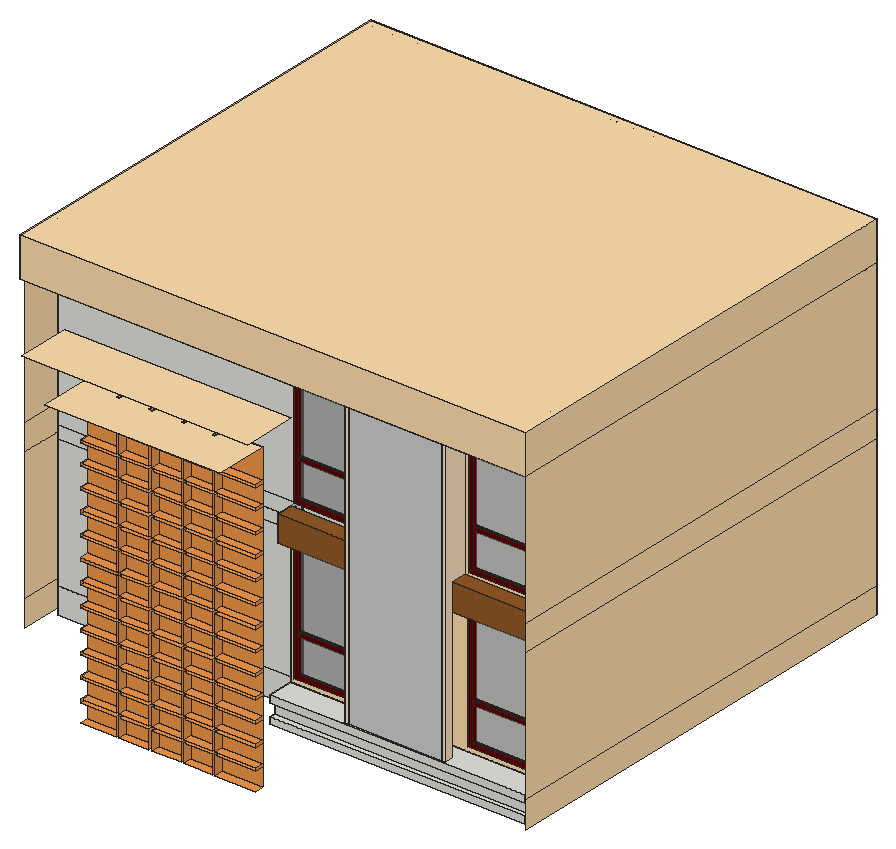
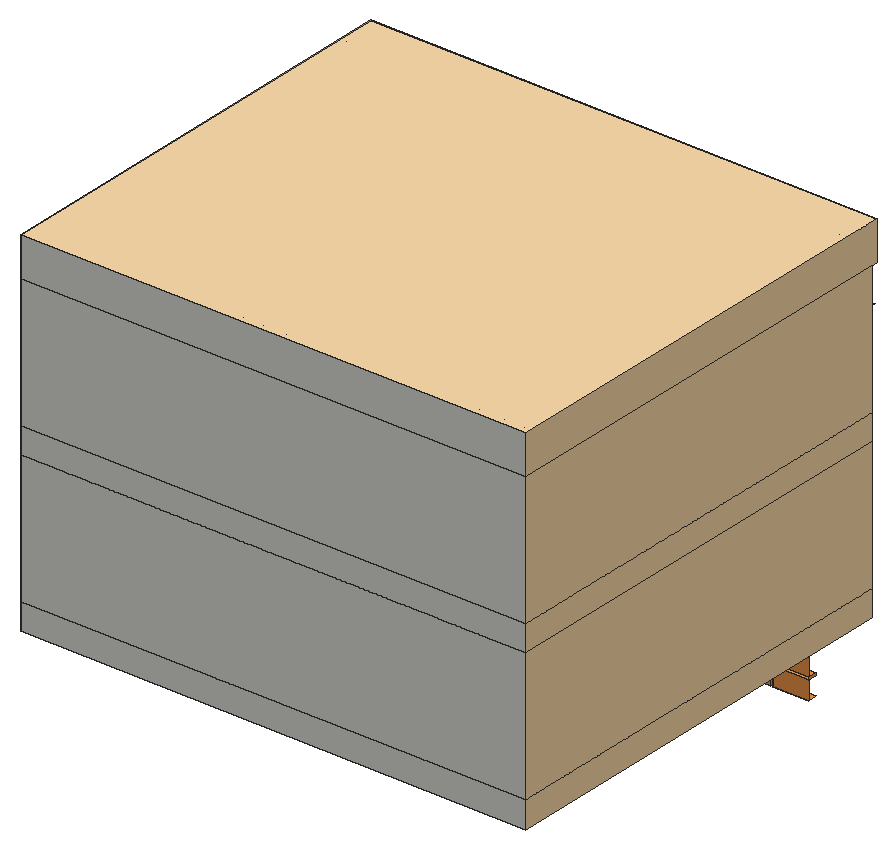
# SketchUp Ruby script. Lengths in inches.
U = 1.inch
M = Sketchup.active_model
def pt(a) = Geom::Point3d.new(a.map { |v| v * U })
def face(e, loops, mat)
  f = e.add_face(loops[0].map { |a| pt(a) })
  loops[1..].each { |l| e.add_face(l.map { |a| pt(a) }).erase! }
  f.material = f.back_material = mat if mat
  f
end
# faces: each face lists its corners as indices into pts; further lists are holes
def faces(e, pts, list, mat = nil) = list.each { |f| face(e, (f[0].is_a?(Array) ? f : [f]).map { |l| l.map { |i| pts[i] } }, mat) }
# xy, xz, yz: faces in a plane at the given z, y or x. An outline is a flat list of corners, or four numbers for a rectangle; further outlines are holes
def ring(l) = l.size == 4 ? [[l[0], l[1]], [l[2], l[1]], [l[2], l[3]], [l[0], l[3]]] : l.each_slice(2).to_a
def flat(e, list, mat, &to3) = list.each { |f| face(e, (f[0].is_a?(Array) ? f : [f]).map { |l| ring(l).map { |u, v| to3.(u, v) } }, mat) }
def xy(e, z, list, mat = nil) = flat(e, list, mat) { |x, y| [x, y, z] }
def xz(e, y, list, mat = nil) = flat(e, list, mat) { |x, z| [x, y, z] }
def yz(e, x, list, mat = nil) = flat(e, list, mat) { |y, z| [x, y, z] }
def lines(e, pts, list) = list.each { |a, b| e.add_line(pt(pts[a]), pt(pts[b])) }
# prism: a flat outline (further loops are holes) pulled along v
def prism(e, loops, v, mat = nil)
  f = face(e, loops, mat); d = Geom::Vector3d.new(v.map { |x| x * U })
  f.pushpull(f.normal.samedirection?(d) ? d.length : -d.length)
end
def box(e, o, s, mat = nil) = prism(e, [[o, [o[0] + s[0], o[1], o[2]], [o[0] + s[0], o[1] + s[1], o[2]], [o[0], o[1] + s[1], o[2]]]], [0, 0, s[2]], mat)
def at(x, y, z, deg = 0) = Geom::Transformation.translation(pt([x, y, z])) * Geom::Transformation.rotation(ORIGIN, Z_AXIS, deg.degrees)
def axes(o, x, y, z) = Geom::Transformation.new([*x, 0, *y, 0, *z, 0, *pt(o).to_a, 1])
def part(name) = M.definitions.add(name)
# library, detail: a bought-in or finely detailed component or shape, given as its bounding box
def library(name, o, s) = part(name).tap { |d| box(d.entities, o, s) }
def detail(e, o, s) = box(e.add_group.entities, o, s)
def put(e, d, t, mat = nil) = e.add_instance(d, t).tap { |i| i.material = mat if mat }
def group(e, t, mat = nil) = e.add_group.tap { |g| g.transformation = t; g.material = mat if mat }.entities
root = M.entities
M.materials.add("[0012_Bisque]").color = [255, 228, 196]
M.materials.add("[0033_NavajoWhite]").color = [255, 222, 173]
M.materials.add("[Carrera Marble]").color = [207, 207, 207]
M.materials.add("[Color A08]").color = [102, 0, 0]
M.materials.add("[Translucent Glass Gray]").color = [128, 128, 128]
M.materials["[Translucent Glass Gray]"].alpha = 0.5
M.materials.add("[Wood Floor Parquet]").color = [145, 89, 39]
M.materials.add("[Wood OSB]").color = [240, 151, 74]
c1 = part("Group\#2")
xy(c1.entities,0,[[0,0,28.5,3]],"[Color A08]")
xy(c1.entities,1.97,[[1.97,0,26.53,3]],"[Color A08]")
xy(c1.entities,16.48,[[1.97,0,26.53,3]],"[Color A08]")
xy(c1.entities,17.92,[[1.97,0,26.53,3]],"[Color A08]")
xy(c1.entities,49.78,[[1.97,0,26.53,3]],"[Color A08]")
xy(c1.entities,51.75,[[0,0,28.5,3]],"[Color A08]")
xz(c1.entities,0,[[[0,0,28.5,51.75],[1.97,1.97,1.97,49.78,26.53,49.78,26.53,17.92,1.97,17.92,1.97,16.48,26.53,16.48,26.53,1.97]]],"[Color A08]")
xz(c1.entities,3,[[[0,0,28.5,51.75],[1.97,1.97,26.53,1.97,26.53,16.48,1.97,16.48,1.97,17.92,26.53,17.92,26.53,49.78,1.97,49.78]]],"[Color A08]")
xz(c1.entities,3,[[1.97,1.97,26.53,16.48],[1.97,17.92,26.53,49.78]],"[Translucent Glass Gray]")
yz(c1.entities,0,[[0,0,3,51.75]],"[Color A08]")
yz(c1.entities,1.97,[[0,1.97,3,16.48],[0,16.48,3,17.92],[0,17.92,3,49.78]],"[Color A08]")
yz(c1.entities,26.53,[[0,1.97,3,16.48],[0,17.92,3,49.78]],"[Color A08]")
yz(c1.entities,28.5,[[0,0,3,51.75]],"[Color A08]")
xy(root,355.36,[[104.2,92.4375,136.74,100.4375],[139.19,92.4375,165.875,100.4375],[169.17,92.4375,195.99,100.4375],[198.13,92.4375,224.24,100.4375],[226.62,92.4375,263.87,100.4375]],"[Wood OSB]")
xy(root,372.03,[[104.2,92.4375,136.74,100.4375],[139.19,92.4375,165.875,100.4375],[169.17,92.4375,195.99,100.4375],[198.13,92.4375,224.24,100.4375],[226.62,92.4375,263.87,100.4375]],"[Wood OSB]")
xy(root,374.67,[[104.2,92.4375,136.74,100.4375],[139.19,92.4375,165.875,100.4375],[169.17,92.4375,195.99,100.4375],[198.13,92.4375,224.24,100.4375],[226.62,92.4375,263.87,100.4375]],"[Wood OSB]")
xy(root,391.34,[[104.2,92.4375,136.74,100.4375],[139.19,92.4375,165.875,100.4375],[169.17,92.4375,195.99,100.4375],[198.13,92.4375,224.24,100.4375],[226.62,92.4375,263.87,100.4375]],"[Wood OSB]")
xy(root,393.98,[[104.2,92.4375,136.74,100.4375],[139.19,92.4375,165.875,100.4375],[169.17,92.4375,195.99,100.4375],[198.13,92.4375,224.24,100.4375],[226.62,92.4375,263.87,100.4375]],"[Wood OSB]")
xy(root,410.65,[[104.2,92.4375,136.74,100.4375],[139.19,92.4375,165.875,100.4375],[169.17,92.4375,195.99,100.4375],[198.13,92.4375,224.24,100.4375],[226.62,92.4375,263.87,100.4375]],"[Wood OSB]")
xy(root,413.3,[[104.2,92.4375,136.74,100.4375],[139.19,92.4375,165.875,100.4375],[169.17,92.4375,195.99,100.4375],[198.13,92.4375,224.24,100.4375],[226.62,92.4375,263.87,100.4375]],"[Wood OSB]")
xy(root,419.04,[[302.01,100.4375,501.57,106.4375]])
xy(root,424.5,[[295.25,106.4375,521.3125,465.125]])
xy(root,426.125,[[289.0625,77,521.3125,100.4375]])
xy(root,429.97,[[104.2,92.4375,136.74,100.4375],[139.19,92.4375,165.875,100.4375],[169.17,92.4375,195.99,100.4375],[198.13,92.4375,224.24,100.4375],[226.62,92.4375,263.87,100.4375]],"[Wood OSB]")
xy(root,432.1875,[[289.0625,77,521.3125,82.1875],[289.0625,82.1875,521.3125,100.4375]])
xy(root,432.61,[[104.2,92.4375,136.74,100.4375],[139.19,92.4375,165.875,100.4375],[169.17,92.4375,195.99,100.4375],[198.13,92.4375,224.24,100.4375],[226.62,92.4375,263.87,100.4375]],"[Wood OSB]")
xy(root,443.4375,[[289.0625,77,521.3125,82.1875],[289.0625,82.1875,521.3125,100.4375]])
xy(root,449.28,[[104.2,92.4375,136.74,100.4375],[139.19,92.4375,165.875,100.4375],[169.17,92.4375,195.99,100.4375],[198.13,92.4375,224.24,100.4375],[226.62,92.4375,263.87,100.4375]],"[Wood OSB]")
xy(root,450.125,[[289.0625,77,355.82,77,355.82,92.4375,359.53,92.4375,359.53,85.8125,448.02,85.8125,448.02,77,521.3125,77,521.3125,100.4375,289.0625,100.4375],[359.53,77,444.31,78.5625],[359.53,78.5625,444.31,85.8125],[71.75,106.4375,289.0625,465.125],[295.0625,106.4375,295.25,465.125],
  [295.25,106.4375,521.3125,465.125]])
xy(root,450.125,[[355.82,77,359.53,78.5625],[444.31,77,448.02,78.5625],[444.31,78.5625,448.02,85.8125]],"[0012_Bisque]")
xy(root,451.92,[[104.2,92.4375,136.74,100.4375],[139.19,92.4375,165.875,100.4375],[169.17,92.4375,195.99,100.4375],[198.13,92.4375,224.24,100.4375],[226.62,92.4375,263.87,100.4375]],"[Wood OSB]")
xy(root,453.93,[[451.2,100.4375,514.83,106.4375]])
xy(root,453.97,[[291.92,100.4375,351.54,106.4375]])
xy(root,468.59,[[104.2,92.4375,136.74,100.4375],[139.19,92.4375,165.875,100.4375],[169.17,92.4375,195.99,100.4375],[198.13,92.4375,224.24,100.4375],[226.62,92.4375,263.87,100.4375]],"[Wood OSB]")
xy(root,471.23,[[104.2,92.4375,136.74,100.4375],[139.19,92.4375,165.875,100.4375],[169.17,92.4375,195.99,100.4375],[198.13,92.4375,224.24,100.4375],[226.62,92.4375,263.87,100.4375]],"[Wood OSB]")
xy(root,487.9,[[104.2,92.4375,136.74,100.4375],[136.74,92.4375,139.19,100.4375],[139.19,92.4375,165.875,100.4375],[169.17,92.4375,195.99,100.4375],[198.13,92.4375,224.24,100.4375],
  [226.62,92.4375,263.87,100.4375]],"[Wood OSB]")
xy(root,490.55,[[104.2,92.4375,136.74,100.4375],[136.74,92.4375,139.19,100.4375],[139.19,92.4375,165.875,100.4375],[169.17,92.4375,195.99,100.4375],[198.13,92.4375,224.24,100.4375],
  [226.62,92.4375,263.87,100.4375]],"[Wood OSB]")
xy(root,507.22,[[104.2,92.4375,136.74,100.4375],[139.19,92.4375,165.875,100.4375],[169.17,92.4375,195.99,100.4375],[198.13,92.4375,224.24,100.4375],[226.62,92.4375,263.87,100.4375]],"[Wood OSB]")
xy(root,509.86,[[104.2,92.4375,136.74,100.4375],[139.19,92.4375,165.875,100.4375],[169.17,92.4375,195.99,100.4375],[198.13,92.4375,224.24,100.4375],[226.62,92.4375,263.87,100.4375]],"[Wood OSB]")
xy(root,526.53,[[104.2,92.4375,136.74,100.4375],[139.19,92.4375,165.875,100.4375],[169.17,92.4375,195.99,100.4375],[198.13,92.4375,224.24,100.4375],[226.62,92.4375,263.87,100.4375]],"[Wood OSB]")
xy(root,529.17,[[104.2,92.4375,136.74,100.4375],[139.19,92.4375,165.875,100.4375],[169.17,92.4375,195.99,100.4375],[198.13,92.4375,224.24,100.4375],[226.62,92.4375,263.87,100.4375]],"[Wood OSB]")
xy(root,545.84,[[104.2,92.4375,136.74,100.4375],[139.19,92.4375,165.875,100.4375],[169.17,92.4375,195.99,100.4375],[198.13,92.4375,224.24,100.4375],[226.62,92.4375,263.87,100.4375]],"[Wood OSB]")
xy(root,548.48,[[104.2,92.4375,136.74,100.4375],[139.19,92.4375,165.875,100.4375],[169.17,92.4375,195.99,100.4375],[198.13,92.4375,224.24,100.4375],[226.62,92.4375,263.87,100.4375]],"[Wood OSB]")
xy(root,565.15,[[104.2,92.4375,136.74,100.4375],[139.19,92.4375,165.875,100.4375],[169.17,92.4375,195.99,100.4375],[198.13,92.4375,224.24,100.4375],[226.62,92.4375,263.87,100.4375]],"[Wood OSB]")
xy(root,566.47,[[291.92,100.4375,351.54,106.4375]])
xy(root,567.56,[[451.2,100.4375,514.83,106.4375]])
xy(root,567.8,[[104.2,92.4375,136.74,100.4375],[139.19,92.4375,165.875,100.4375],[169.17,92.4375,195.99,100.4375],[198.13,92.4375,224.24,100.4375],[226.62,92.4375,263.87,100.4375]],"[Wood OSB]")
xy(root,570.125,[[295.0625,106.4375,295.25,465.125]])
xy(root,570.125,[[355.82,85.8125,359.53,92.4375]],"[0012_Bisque]")
xy(root,570.125,[[289.0625,85.8125,289.0625,100.4375,521.3125,100.4375,521.3125,85.8125,359.53,85.8125,359.53,92.4375,355.82,92.4375,355.82,85.8125]],"[Wood Floor Parquet]")
xy(root,581.3125,[[71.75,106.4375,289.0625,465.125]])
xy(root,584.47,[[104.2,92.4375,136.74,100.4375],[139.19,92.4375,165.875,100.4375],[169.17,92.4375,195.99,100.4375],[198.13,92.4375,224.24,100.4375],[226.62,92.4375,263.87,100.4375]],"[Wood OSB]")
xy(root,587.11,[[104.2,92.4375,136.74,100.4375],[139.19,92.4375,165.875,100.4375],[169.17,92.4375,195.99,100.4375],[198.13,92.4375,224.24,100.4375],[226.62,92.4375,263.87,100.4375]],"[Wood OSB]")
xy(root,594.125,[[71.75,106.4375,289.0625,465.125],[295.0625,106.4375,521.3125,465.125]])
xy(root,594.125,[[289.0625,85.8125,355.82,100.4375],[355.82,85.8125,359.53,100.4375],[359.53,85.8125,444.31,100.4375],[444.31,85.8125,448.02,100.4375],[448.02,85.8125,521.3125,100.4375]],"[Wood Floor Parquet]")
xy(root,596.59,[[451.48,100.4375,515.23,106.4375]])
xy(root,597.4375,[[292.08,100.4375,351.27,106.4375]])
xy(root,603.78,[[104.2,92.4375,136.74,100.4375],[139.19,92.4375,165.875,100.4375],[169.17,92.4375,195.99,100.4375],[198.13,92.4375,224.24,100.4375],[226.62,92.4375,263.87,100.4375]],"[Wood OSB]")
xy(root,606.42,[[104.2,92.4375,136.74,100.4375],[139.19,92.4375,165.875,100.4375],[169.17,92.4375,195.99,100.4375],[198.13,92.4375,224.24,100.4375],[226.62,92.4375,263.87,100.4375]],"[Wood OSB]")
xy(root,633.42,[[104.2,51.6875,104.2,100.4375,136.74,100.4375,136.74,92.4375,139.19,92.4375,139.19,100.4375,165.875,100.4375,165.875,92.4375,169.17,92.4375,169.17,100.4375,195.99,100.4375,195.99,92.4375,198.13,92.4375,198.13,100.4375,224.24,100.4375,224.24,92.4375,226.62,92.4375,226.62,100.4375,263.87,100.4375,263.87,51.6875]],"[0033_NavajoWhite]")
xy(root,633.42,[[136.74,92.4375,139.19,100.4375],[165.875,92.4375,169.17,100.4375],[195.99,92.4375,198.13,100.4375],[224.24,92.4375,226.62,100.4375]],"[Wood OSB]")
xy(root,665.86,[[82.77,51.6875,289.0625,100.4375]],"[0033_NavajoWhite]")
xy(root,710.4,[[359.53,78.5625,444.31,100.4375]])
xy(root,711.0625,[[292.08,100.4375,351.27,106.4375]])
xy(root,711.15,[[451.48,100.4375,515.23,106.4375]])
xy(root,714.125,[[[521.3125,71.3125,521.3125,100.4375,289.0625,100.4375,289.0625,465.125,71.75,465.125,71.75,106.4375,289.0625,106.4375,289.0625,100.4375,71.75,100.4375,71.75,77,65.75,77,65.75,471.125,527.3125,471.125,527.3125,71.3125],[295.0625,106.4375,521.3125,465.125]]])
xy(root,714.125,[[355.82,78.5625,448.02,100.4375]],"[0012_Bisque]")
xy(root,714.125,[[65.75,71.3125,65.75,77,71.75,77,71.75,100.4375,355.82,100.4375,355.82,78.5625,448.02,78.5625,448.02,100.4375,521.3125,100.4375,521.3125,71.3125]],"[0033_NavajoWhite]")
xy(root,745.125,[[71.75,106.4375,289.0625,465.125],[295.0625,106.4375,521.3125,465.125]])
xy(root,750.125,[[65.75,71.3125,527.3125,471.125]],"[0033_NavajoWhite]")
xz(root,71.3125,[[65.75,714.125,527.3125,750.125]],"[0033_NavajoWhite]")
xz(root,77,[[289.0625,426.125,521.3125,432.1875],[289.0625,443.4375,521.3125,450.125]])
xz(root,78.5625,[[355.82,450.125,359.53,450.125,359.53,710.4,444.31,710.4,444.31,450.125,448.02,450.125,448.02,714.125,355.82,714.125]],"[0012_Bisque]")
xz(root,78.5625,[[359.53,450.125,444.31,710.4]],"[Carrera Marble]")
xz(root,82.1875,[[289.0625,432.1875,521.3125,443.4375]])
xz(root,85.8125,[[359.53,450.125,444.31,570.125],[359.53,570.125,444.31,594.125]])
xz(root,85.8125,[[444.31,450.125,448.02,570.125]],"[0012_Bisque]")
xz(root,85.8125,[[289.0625,570.125,355.82,594.125],[355.82,570.125,359.53,594.125],[444.31,570.125,448.02,594.125],[448.02,570.125,521.3125,594.125]],"[Wood Floor Parquet]")
xz(root,92.4375,[[355.82,450.125,359.53,570.125]],"[0012_Bisque]")
xz(root,92.4375,[[104.2,487.9,139.19,490.55]],"[Wood OSB]")
xz(root,100.4375,[[289.0625,426.125,521.3125,432.1875],[289.0625,443.4375,521.3125,450.125],[355.82,590.41,448.02,594.125],[355.82,714.125,448.02,717.84]])
xz(root,100.4375,[[355.82,594.125,355.82,714.125,448.02,714.125,448.02,594.125,444.31,594.125,444.31,710.4,359.53,710.4,359.53,594.125]],"[0012_Bisque]")
xz(root,100.4375,[[[289.0625,450.125,521.3125,570.125],[451.2,453.93,514.83,567.56],[291.92,453.97,351.54,566.47]],[[448.02,594.125,521.3125,714.125],[451.48,596.59,515.23,711.15]]],"[0033_NavajoWhite]")
xz(root,100.4375,[[104.2,355.36,136.74,372.03],[139.19,355.36,165.875,372.03],[169.17,355.36,195.99,372.03],[198.13,355.36,224.24,372.03],[226.62,355.36,263.87,372.03],
  [104.2,374.67,136.74,391.34],[139.19,374.67,165.875,391.34],[169.17,374.67,195.99,391.34],[198.13,374.67,224.24,391.34],[226.62,374.67,263.87,391.34],
  [104.2,393.98,136.74,410.65],[139.19,393.98,165.875,410.65],[169.17,393.98,195.99,410.65],[198.13,393.98,224.24,410.65],[226.62,393.98,263.87,410.65],
  [104.2,413.3,136.74,429.97],[139.19,413.3,165.875,429.97],[169.17,413.3,195.99,429.97],[198.13,413.3,224.24,429.97],[226.62,413.3,263.87,429.97],
  [104.2,432.61,136.74,449.28],[139.19,432.61,165.875,449.28],[169.17,432.61,195.99,449.28],[198.13,432.61,224.24,449.28],[226.62,432.61,263.87,449.28],
  [104.2,451.92,136.74,468.59],[139.19,451.92,165.875,468.59],[169.17,451.92,195.99,468.59],[198.13,451.92,224.24,468.59],[226.62,451.92,263.87,468.59],
  [104.2,471.23,136.74,487.9],[139.19,471.23,165.875,487.9],[169.17,471.23,195.99,487.9],[198.13,471.23,224.24,487.9],[226.62,471.23,263.87,487.9],
  [104.2,490.55,136.74,507.22],[139.19,490.55,165.875,507.22],[169.17,490.55,195.99,507.22],[198.13,490.55,224.24,507.22],[226.62,490.55,263.87,507.22],
  [104.2,509.86,136.74,526.53],[139.19,509.86,165.875,526.53],[169.17,509.86,195.99,526.53],[198.13,509.86,224.24,526.53],[226.62,509.86,263.87,526.53],
  [104.2,529.17,136.74,545.84],[139.19,529.17,165.875,545.84],[169.17,529.17,195.99,545.84],[198.13,529.17,224.24,545.84],[226.62,529.17,263.87,545.84],
  [104.2,548.48,136.74,565.15],[139.19,548.48,165.875,565.15],[169.17,548.48,195.99,565.15],[198.13,548.48,224.24,565.15],[226.62,548.48,263.87,565.15],
  [104.2,567.8,136.74,584.47],[139.19,567.8,165.875,584.47],[169.17,567.8,195.99,584.47],[198.13,567.8,224.24,584.47],[226.62,567.8,263.87,584.47],
  [104.2,587.11,136.74,603.78],[139.19,587.11,165.875,603.78],[169.17,587.11,195.99,603.78],[198.13,587.11,224.24,603.78],[226.62,587.11,263.87,603.78],
  [104.2,606.42,136.74,633.42],[139.19,606.42,165.875,633.42],[169.17,606.42,195.99,633.42],[198.13,606.42,224.24,633.42],[226.62,606.42,263.87,633.42]],"[Wood OSB]")
xz(root,106.4375,[[295.25,424.5,384.66,426.125],[384.66,424.5,387.91,426.125],[384.66,424.5,387.91,426.125],[387.91,424.5,521.3125,426.125],[71.75,426.125,289.0625,450.125],
  [295.0625,426.125,295.25,450.125],[295.25,426.125,384.66,450.125],[384.66,426.125,387.91,450.125],[387.91,426.125,521.3125,450.125],[71.75,450.125,289.0625,570.125],
  [295.0625,450.125,295.25,453.97],[[295.25,450.125,295.25,453.97,351.54,453.97,351.54,566.47,295.25,566.47,295.25,570.125,521.3125,570.125,521.3125,450.125],[451.2,453.93,514.83,567.56]],[291.92,453.97,295.0625,566.47],[295.0625,453.97,295.25,566.47],[295.25,453.97,351.54,566.47],
  [295.0625,566.47,295.25,570.125],[71.75,570.125,289.0625,581.3125],[295.0625,570.125,295.25,594.125],[295.25,570.125,521.3125,594.125],[71.75,581.3125,289.0625,594.125],
  [71.75,594.125,289.0625,714.125],[295.0625,594.125,295.25,597.4375],[[295.25,594.125,295.25,597.4375,351.27,597.4375,351.27,711.0625,295.25,711.0625,295.25,714.125,521.3125,714.125,521.3125,594.125],[451.48,596.59,515.23,711.15]],[292.08,597.4375,295.0625,711.0625],[295.0625,597.4375,295.25,711.0625],
  [295.25,597.4375,351.27,711.0625],[295.0625,711.0625,295.25,714.125]])
xz(root,465.125,[[295.25,424.5,521.3125,426.125],[71.75,426.125,289.0625,450.125],[295.0625,426.125,295.25,450.125],[295.25,426.125,521.3125,450.125],[71.75,450.125,289.0625,570.125],
  [295.0625,450.125,295.25,570.125],[295.25,450.125,521.3125,570.125],[71.75,570.125,289.0625,581.3125],[295.0625,570.125,295.25,594.125],[295.25,570.125,521.3125,594.125],
  [71.75,581.3125,80.67,594.125],[80.67,581.3125,84.35,594.125],[84.35,581.3125,87.92,594.125],[87.92,581.3125,289.0625,594.125],[71.75,594.125,289.0625,714.125],
  [295.0625,594.125,295.25,714.125],[295.25,594.125,521.3125,714.125],[71.75,714.125,289.0625,745.125],[295.0625,714.125,295.25,745.125],[295.25,714.125,521.3125,745.125],
  [295.0625,745.125,295.25,750.125]])
xz(root,471.125,[[65.75,426.125,527.3125,450.125],[65.75,450.125,527.3125,570.125],[65.75,570.125,527.3125,594.125],[65.75,594.125,527.3125,714.125],[65.75,714.125,527.3125,750.125]])
yz(root,65.75,[[77,426.125,471.125,450.125],[77,450.125,471.125,570.125],[77,570.125,471.125,594.125],[77,594.125,471.125,714.125],[71.3125,714.125,471.125,750.125]],"[0033_NavajoWhite]")
yz(root,71.75,[[106.4375,426.125,465.125,450.125],[106.4375,450.125,465.125,570.125],[106.4375,570.125,465.125,581.3125],[106.4375,581.3125,465.125,594.125],[106.4375,594.125,465.125,714.125],
  [106.4375,714.125,465.125,745.125]])
yz(root,104.2,[[92.4375,372.03,100.4375,374.67],[92.4375,391.34,100.4375,393.98],[92.4375,410.65,100.4375,413.3],[92.4375,429.97,100.4375,432.61],[92.4375,449.28,100.4375,451.92],
  [92.4375,468.59,100.4375,471.23],[92.4375,507.22,100.4375,509.86],[92.4375,526.53,100.4375,529.17],[92.4375,545.84,100.4375,548.48],[92.4375,565.15,100.4375,567.8],
  [92.4375,584.47,100.4375,587.11],[92.4375,603.78,100.4375,606.42]],"[Wood OSB]")
yz(root,136.74,[[92.4375,355.36,100.4375,372.03],[92.4375,374.67,100.4375,391.34],[92.4375,393.98,100.4375,410.65],[92.4375,413.3,100.4375,429.97],[92.4375,432.61,100.4375,449.28],
  [92.4375,451.92,100.4375,468.59],[92.4375,471.23,100.4375,487.9],[92.4375,490.55,100.4375,507.22],[92.4375,509.86,100.4375,526.53],[92.4375,529.17,100.4375,545.84],
  [92.4375,548.48,100.4375,565.15],[92.4375,567.8,100.4375,584.47],[92.4375,587.11,100.4375,603.78],[92.4375,606.42,100.4375,633.42]],"[Wood OSB]")
yz(root,139.19,[[92.4375,355.36,100.4375,372.03],[92.4375,374.67,100.4375,391.34],[92.4375,393.98,100.4375,410.65],[92.4375,413.3,100.4375,429.97],[92.4375,432.61,100.4375,449.28],
  [92.4375,451.92,100.4375,468.59],[92.4375,471.23,100.4375,487.9],[92.4375,487.9,100.4375,490.55],[92.4375,490.55,100.4375,507.22],[92.4375,509.86,100.4375,526.53],
  [92.4375,529.17,100.4375,545.84],[92.4375,548.48,100.4375,565.15],[92.4375,567.8,100.4375,584.47],[92.4375,587.11,100.4375,603.78],[92.4375,606.42,100.4375,633.42]],"[Wood OSB]")
yz(root,165.875,[[92.4375,355.36,100.4375,372.03],[92.4375,374.67,100.4375,391.34],[92.4375,393.98,100.4375,410.65],[92.4375,413.3,100.4375,429.97],[92.4375,432.61,100.4375,449.28],
  [92.4375,451.92,100.4375,468.59],[92.4375,471.23,100.4375,487.9],[92.4375,490.55,100.4375,507.22],[92.4375,509.86,100.4375,526.53],[92.4375,529.17,100.4375,545.84],
  [92.4375,548.48,100.4375,565.15],[92.4375,567.8,100.4375,584.47],[92.4375,587.11,100.4375,603.78],[92.4375,606.42,100.4375,633.42]],"[Wood OSB]")
yz(root,169.17,[[92.4375,355.36,100.4375,372.03],[92.4375,374.67,100.4375,391.34],[92.4375,393.98,100.4375,410.65],[92.4375,413.3,100.4375,429.97],[92.4375,432.61,100.4375,449.28],
  [92.4375,451.92,100.4375,468.59],[92.4375,471.23,100.4375,487.9],[92.4375,490.55,100.4375,507.22],[92.4375,509.86,100.4375,526.53],[92.4375,529.17,100.4375,545.84],
  [92.4375,548.48,100.4375,565.15],[92.4375,567.8,100.4375,584.47],[92.4375,587.11,100.4375,603.78],[92.4375,606.42,100.4375,633.42]],"[Wood OSB]")
yz(root,195.99,[[92.4375,355.36,100.4375,372.03],[92.4375,374.67,100.4375,391.34],[92.4375,393.98,100.4375,410.65],[92.4375,413.3,100.4375,429.97],[92.4375,432.61,100.4375,449.28],
  [92.4375,451.92,100.4375,468.59],[92.4375,471.23,100.4375,487.9],[92.4375,490.55,100.4375,507.22],[92.4375,509.86,100.4375,526.53],[92.4375,529.17,100.4375,545.84],
  [92.4375,548.48,100.4375,565.15],[92.4375,567.8,100.4375,584.47],[92.4375,587.11,100.4375,603.78],[92.4375,606.42,100.4375,633.42]],"[Wood OSB]")
yz(root,198.13,[[92.4375,355.36,100.4375,372.03],[92.4375,374.67,100.4375,391.34],[92.4375,393.98,100.4375,410.65],[92.4375,413.3,100.4375,429.97],[92.4375,432.61,100.4375,449.28],
  [92.4375,451.92,100.4375,468.59],[92.4375,471.23,100.4375,487.9],[92.4375,490.55,100.4375,507.22],[92.4375,509.86,100.4375,526.53],[92.4375,529.17,100.4375,545.84],
  [92.4375,548.48,100.4375,565.15],[92.4375,567.8,100.4375,584.47],[92.4375,587.11,100.4375,603.78],[92.4375,606.42,100.4375,633.42]],"[Wood OSB]")
yz(root,224.24,[[92.4375,355.36,100.4375,372.03],[92.4375,374.67,100.4375,391.34],[92.4375,393.98,100.4375,410.65],[92.4375,413.3,100.4375,429.97],[92.4375,432.61,100.4375,449.28],
  [92.4375,451.92,100.4375,468.59],[92.4375,471.23,100.4375,487.9],[92.4375,490.55,100.4375,507.22],[92.4375,509.86,100.4375,526.53],[92.4375,529.17,100.4375,545.84],
  [92.4375,548.48,100.4375,565.15],[92.4375,567.8,100.4375,584.47],[92.4375,587.11,100.4375,603.78],[92.4375,606.42,100.4375,633.42]],"[Wood OSB]")
yz(root,226.62,[[92.4375,355.36,100.4375,372.03],[92.4375,374.67,100.4375,391.34],[92.4375,393.98,100.4375,410.65],[92.4375,413.3,100.4375,429.97],[92.4375,432.61,100.4375,449.28],
  [92.4375,451.92,100.4375,468.59],[92.4375,471.23,100.4375,487.9],[92.4375,490.55,100.4375,507.22],[92.4375,509.86,100.4375,526.53],[92.4375,529.17,100.4375,545.84],
  [92.4375,548.48,100.4375,565.15],[92.4375,567.8,100.4375,584.47],[92.4375,587.11,100.4375,603.78],[92.4375,606.42,100.4375,633.42]],"[Wood OSB]")
yz(root,263.87,[[92.4375,372.03,100.4375,374.67],[92.4375,391.34,100.4375,393.98],[92.4375,410.65,100.4375,413.3],[92.4375,429.97,100.4375,432.61],[92.4375,449.28,100.4375,451.92],
  [92.4375,468.59,100.4375,471.23],[92.4375,487.9,100.4375,490.55],[92.4375,507.22,100.4375,509.86],[92.4375,526.53,100.4375,529.17],[92.4375,545.84,100.4375,548.48],
  [92.4375,565.15,100.4375,567.8],[92.4375,584.47,100.4375,587.11],[92.4375,603.78,100.4375,606.42]],"[Wood OSB]")
yz(root,289.0625,[[77,426.125,100.4375,432.1875],[100.4375,426.125,100.4375,432.1875,82.1875,432.1875,82.1875,443.4375,100.4375,443.4375,100.4375,450.125,106.4375,450.125,106.4375,426.125],[106.4375,426.125,465.125,450.125],[77,443.4375,100.4375,450.125],[100.4375,450.125,106.4375,570.125],
  [106.4375,450.125,465.125,570.125],[85.8125,570.125,106.4375,594.125],[106.4375,570.125,465.125,581.3125],[106.4375,581.3125,465.125,594.125],[106.4375,594.125,465.125,714.125]])
yz(root,291.92,[[100.4375,453.97,106.4375,566.47]])
yz(root,292.08,[[100.4375,597.4375,106.4375,711.0625]])
yz(root,295.0625,[[106.4375,426.125,465.125,450.125],[106.4375,450.125,465.125,570.125],[106.4375,570.125,465.125,594.125],[106.4375,594.125,465.125,714.125]])
yz(root,295.25,[[106.4375,424.5,465.125,450.125],[106.4375,450.125,465.125,570.125]])
yz(root,351.27,[[100.4375,597.4375,106.4375,711.0625]])
yz(root,351.54,[[100.4375,453.97,106.4375,566.47]])
yz(root,355.82,[[78.5625,450.125,78.5625,714.125,100.4375,714.125,100.4375,594.125,85.8125,594.125,85.8125,570.125,92.4375,570.125,92.4375,450.125]],"[0012_Bisque]")
yz(root,359.53,[[78.5625,450.125,85.8125,450.125,85.8125,594.125,100.4375,594.125,100.4375,710.4,78.5625,710.4]])
yz(root,359.53,[[85.8125,450.125,92.4375,468.3125],[85.8125,468.3125,92.4375,570.125]],"[0012_Bisque]")
yz(root,444.31,[[78.5625,450.125,78.5625,710.4,100.4375,710.4,100.4375,594.125,85.8125,594.125,85.8125,450.125]])
yz(root,448.02,[[78.5625,450.125,85.8125,450.125,85.8125,594.125,100.4375,594.125,100.4375,714.125,78.5625,714.125]],"[0012_Bisque]")
yz(root,451.2,[[100.4375,453.93,106.4375,567.56]])
yz(root,451.48,[[100.4375,596.59,106.4375,711.15]])
yz(root,514.83,[[100.4375,453.93,106.4375,567.56]])
yz(root,515.23,[[100.4375,596.59,106.4375,711.15]])
yz(root,521.3125,[[106.4375,424.5,465.125,426.125],[77,426.125,100.4375,432.1875],[106.4375,426.125,465.125,450.125],[77,443.4375,100.4375,450.125],[106.4375,450.125,465.125,570.125],
  [106.4375,570.125,465.125,594.125],[106.4375,594.125,465.125,714.125],[106.4375,714.125,465.125,745.125]])
yz(root,527.3125,[[71.3125,426.125,471.125,450.125],[71.3125,450.125,471.125,570.125],[71.3125,570.125,471.125,594.125],[71.3125,594.125,471.125,714.125],[71.3125,714.125,471.125,750.125]],"[0033_NavajoWhite]")
p = [[90.375,465.125,750.125],[90.375,465.125,745.125],[112.875,465.125,750.125],[112.875,465.125,745.125],[71.75,106.4375,745.125],[71.75,106.4375,750.125],
  [71.75,465.125,745.125],[71.75,465.125,750.125],[289.0625,465.125,745.125],[289.0625,465.125,750.125],[310.01,465.125,750.125],[310.01,465.125,745.125],
  [328.39,465.125,750.125],[328.39,465.125,745.125],[521.3125,106.4375,745.125],[521.3125,106.4375,750.125]]
lines(root,p,[[0,1],[2,3],[4,5],[6,7],[8,9],[10,11],[12,13],[14,15]])
put(root,c1,axes([292.19,100.71,453.93],[2.08238,0,0],[0,0.91,0],[0,0,2.1747]))
put(root,c1,axes([451.2,100.4375,453.93],[2.23246,0,0],[0,1,0],[0,0,2.19565]))
put(root,c1,axes([451.6,100.4375,596.59],[2.23246,0,0],[0,1,0],[0,0,2.19565]))
put(root,c1,axes([291.92,100.71,597.4],[2.08238,0,0],[0,0.91,0],[0,0,2.1747]))
